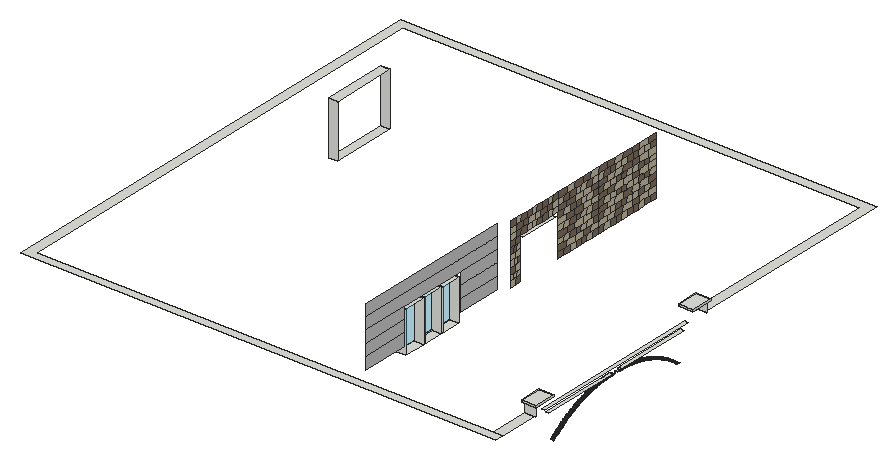
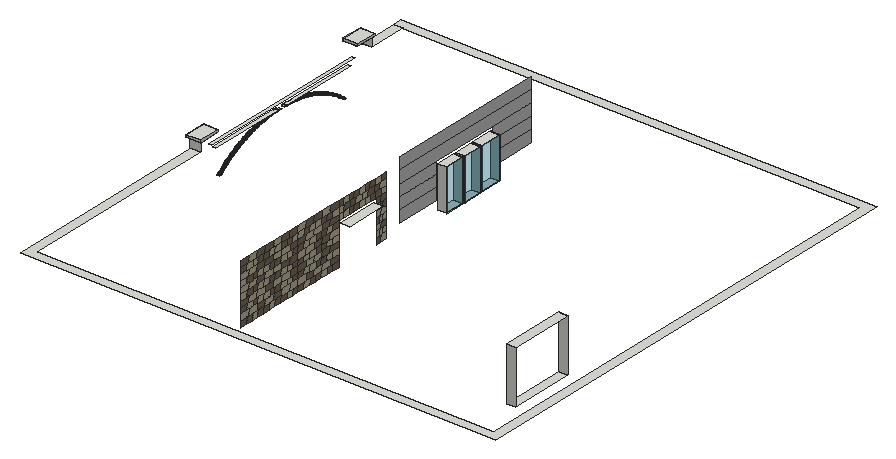
# SketchUp Ruby script. Lengths in inches.
U = 1.inch
M = Sketchup.active_model
def pt(a) = Geom::Point3d.new(a.map { |v| v * U })
def face(e, loops, mat)
  f = e.add_face(loops[0].map { |a| pt(a) })
  loops[1..].each { |l| e.add_face(l.map { |a| pt(a) }).erase! }
  f.material = f.back_material = mat if mat
  f
end
# faces: each face lists its corners as indices into pts; further lists are holes
def faces(e, pts, list, mat = nil) = list.each { |f| face(e, (f[0].is_a?(Array) ? f : [f]).map { |l| l.map { |i| pts[i] } }, mat) }
# xy, xz, yz: faces in a plane at the given z, y or x. An outline is a flat list of corners, or four numbers for a rectangle; further outlines are holes
def ring(l) = l.size == 4 ? [[l[0], l[1]], [l[2], l[1]], [l[2], l[3]], [l[0], l[3]]] : l.each_slice(2).to_a
def flat(e, list, mat, &to3) = list.each { |f| face(e, (f[0].is_a?(Array) ? f : [f]).map { |l| ring(l).map { |u, v| to3.(u, v) } }, mat) }
def xy(e, z, list, mat = nil) = flat(e, list, mat) { |x, y| [x, y, z] }
def xz(e, y, list, mat = nil) = flat(e, list, mat) { |x, z| [x, y, z] }
def yz(e, x, list, mat = nil) = flat(e, list, mat) { |y, z| [x, y, z] }
def lines(e, pts, list) = list.each { |a, b| e.add_line(pt(pts[a]), pt(pts[b])) }
# prism: a flat outline (further loops are holes) pulled along v
def prism(e, loops, v, mat = nil)
  f = face(e, loops, mat); d = Geom::Vector3d.new(v.map { |x| x * U })
  f.pushpull(f.normal.samedirection?(d) ? d.length : -d.length)
end
def box(e, o, s, mat = nil) = prism(e, [[o, [o[0] + s[0], o[1], o[2]], [o[0] + s[0], o[1] + s[1], o[2]], [o[0], o[1] + s[1], o[2]]]], [0, 0, s[2]], mat)
def at(x, y, z, deg = 0) = Geom::Transformation.translation(pt([x, y, z])) * Geom::Transformation.rotation(ORIGIN, Z_AXIS, deg.degrees)
def axes(o, x, y, z) = Geom::Transformation.new([*x, 0, *y, 0, *z, 0, *pt(o).to_a, 1])
def part(name) = M.definitions.add(name)
# library, detail: a bought-in or finely detailed component or shape, given as its bounding box
def library(name, o, s) = part(name).tap { |d| box(d.entities, o, s) }
def detail(e, o, s) = box(e.add_group.entities, o, s)
def put(e, d, t, mat = nil) = e.add_instance(d, t).tap { |i| i.material = mat if mat }
def group(e, t, mat = nil) = e.add_group.tap { |g| g.transformation = t; g.material = mat if mat }.entities
root = M.entities
M.materials.add("Brick_05_1K").color = [195, 185, 161]
M.materials.add("Brick_20_1K1").color = [126, 109, 93]
M.materials.add("Glass_Basic_01").color = [33, 150, 186]
M.materials["Glass_Basic_01"].alpha = 0.4
M.materials.add("M02_Ash_Whisper").color = [196, 196, 196]
M.materials.add("ThomThom - Buttons1").color = [48, 49, 53]
xy(root,63,[[294,108,303,130],[57,318,66,384]])
xy(root,86.9,[[474,151,477,153.9],[474,158.1,477,161]])
xy(root,88,[[474,71,477,151],[474,161,477,241]])
xy(root,93,[[474,66,477,246]])
xy(root,96,[[0,0,480,0,480,9,9,9,9,471,471,471,471,264,480,264,480,480,0,480],[471,9,480,48]])
xy(root,105,[[294,108,303,130],[294,255,303,297]])
xy(root,106,[[469,46,484,48],[469,48,471,68],[482,48,484,66],[471,66,480,68],[480,66,484,68],
  [469,244,484,246],[469,246,471,264],[482,246,484,264],[469,264,480,266],[480,264,484,266]])
xy(root,108,[[469,46,484,68],[469,244,484,266]])
xy(root,117,[[57,318,66,384]])
xz(root,46,[[469,106,484,108]])
xz(root,48,[[471,96,482,106]])
xz(root,68,[[469,106,484,108]])
xz(root,108,[[294,63,303,105]])
xz(root,130,[[294,63,303,105]])
xz(root,132.01,[[294,62.88,303,104.88]])
xz(root,152,[[294,63,303,105]])
xz(root,154.01,[[294,62.88,303,104.88]])
xz(root,174,[[294,63,303,105]])
xz(root,244,[[469,106,484,108]])
xz(root,264,[[471,96,482,106]])
xz(root,266,[[469,106,484,108]])
xz(root,318,[[57,63,66,117]])
xz(root,384,[[57,63,66,117]])
yz(root,294,[[132.01,62.88,152,63,152,62.88],[154.01,62.88,174,63,174,62.88],[132.01,104.88,132.01,105,152,105],[154.01,104.88,154.01,105,174,105]])
yz(root,294,[[132.01,62.88,132.01,104.88,152,105,152,63],[154.01,62.88,154.01,104.88,174,105,174,63],[108,63,130,105]],"Glass_Basic_01")
yz(root,303,[[240,66,246,72],[314.47,66,321.71,72],[336.18,66,343.41,72],[357.88,66,365.12,72],[379.59,66,386.82,72],
  [401.29,66,408.53,72],[240,72,244,78],[244,72,248,78],[248,72,252,78],[310.25,72,320.5,78],
  [320.5,72,330.75,78],[341,72,351.25,78],[351.25,72,361.5,78],[361.5,72,371.75,78],[382,72,392.25,78],
  [402.5,72,412.75,78],[412.75,72,423,78],[246,78,252,84],[300,78,307.24,84],[307.24,78,314.47,84],
  [328.94,78,336.18,84],[336.18,78,343.41,84],[357.88,78,365.12,84],[365.12,78,372.35,84],[386.82,78,394.06,84],
  [394.06,78,401.29,84],[408.53,78,415.76,84],[240,84,244,90],[244,84,248,90],[320.5,84,330.75,90],
  [330.75,84,341,90],[361.5,84,371.75,90],[371.75,84,382,90],[392.25,84,402.5,90],[402.5,84,412.75,90],
  [240,90,246,96],[246,90,252,96],[300,90,307.24,96],[307.24,90,314.47,96],[328.94,90,336.18,96],
  [336.18,90,343.41,96],[357.88,90,365.12,96],[365.12,90,372.35,96],[386.82,90,394.06,96],[394.06,90,401.29,96],
  [415.76,90,423,96],[248,96,252,102],[300,96,310.25,102],[330.75,96,341,102],[341,96,351.25,102],
  [371.75,96,382,102],[382,96,392.25,102],[402.5,96,412.75,102],[412.75,96,423,102],[307.24,102,314.47,108],
  [328.94,102,336.18,108],[336.18,102,343.41,108],[357.88,102,365.12,108],[365.12,102,372.35,108],[386.82,102,394.06,108],
  [394.06,102,401.29,108],[415.76,102,423,108],[240,108,246.67,114],[260,108,266.67,114],[266.67,108,273.33,114],
  [286.67,108,293.33,114],[293.33,108,300,114],[320.5,108,330.75,114],[330.75,108,341,114],[361.5,108,371.75,114],
  [371.75,108,382,114],[402.5,108,412.75,114],[412.75,108,423,114],[240,114,247.5,120],[262.5,114,270,120],
  [270,114,277.5,120],[292.5,114,300,120],[300,114,307.24,120],[321.71,114,328.94,120],[328.94,114,336.18,120],
  [343.41,114,350.65,120],[350.65,114,357.88,120],[372.35,114,379.59,120],[379.59,114,386.82,120],[401.29,114,408.53,120],
  [408.53,114,415.76,120],[246.67,120,253.33,126],[266.67,120,273.33,126],[286.67,120,293.33,126],[310.25,120,320.5,126],
  [341,120,351.25,126],[371.75,120,382,126],[402.5,120,412.75,126]],"Brick_05_1K")
yz(root,303,[[246,66,252,72],[300,66,307.24,72],[307.24,66,314.47,72],[321.71,66,328.94,72],[328.94,66,336.18,72],
  [343.41,66,350.65,72],[350.65,66,357.88,72],[365.12,66,372.35,72],[372.35,66,379.59,72],[386.82,66,394.06,72],
  [394.06,66,401.29,72],[408.53,66,415.76,72],[415.76,66,423,72],[300,72,310.25,78],[330.75,72,341,78],
  [371.75,72,382,78],[392.25,72,402.5,78],[240,78,246,84],[314.47,78,321.71,84],[321.71,78,328.94,84],
  [343.41,78,350.65,84],[350.65,78,357.88,84],[372.35,78,379.59,84],[379.59,78,386.82,84],[401.29,78,408.53,84],
  [415.76,78,423,84],[248,84,252,90],[300,84,310.25,90],[310.25,84,320.5,90],[341,84,351.25,90],
  [351.25,84,361.5,90],[382,84,392.25,90],[412.75,84,423,90],[314.47,90,321.71,96],[321.71,90,328.94,96],
  [343.41,90,350.65,96],[350.65,90,357.88,96],[372.35,90,379.59,96],[379.59,90,386.82,96],[401.29,90,408.53,96],
  [408.53,90,415.76,96],[240,96,244,102],[244,96,248,102],[310.25,96,320.5,102],[320.5,96,330.75,102],
  [351.25,96,361.5,102],[361.5,96,371.75,102],[392.25,96,402.5,102],[240,102,246,108],[246,102,252,108],
  [300,102,307.24,108],[314.47,102,321.71,108],[321.71,102,328.94,108],[343.41,102,350.65,108],[350.65,102,357.88,108],
  [372.35,102,379.59,108],[379.59,102,386.82,108],[401.29,102,408.53,108],[408.53,102,415.76,108],[246.67,108,253.33,114],
  [253.33,108,260,114],[273.33,108,280,114],[280,108,286.67,114],[300,108,310.25,114],[310.25,108,320.5,114],
  [341,108,351.25,114],[351.25,108,361.5,114],[382,108,392.25,114],[392.25,108,402.5,114],[247.5,114,255,120],
  [255,114,262.5,120],[277.5,114,285,120],[285,114,292.5,120],[307.24,114,314.47,120],[314.47,114,321.71,120],
  [336.18,114,343.41,120],[357.88,114,365.12,120],[365.12,114,372.35,120],[386.82,114,394.06,120],[394.06,114,401.29,120],
  [415.76,114,423,120],[240,120,246.67,126],[253.33,120,260,126],[260,120,266.67,126],[273.33,120,280,126],
  [280,120,286.67,126],[293.33,120,300,126],[300,120,310.25,126],[320.5,120,330.75,126],[330.75,120,341,126],
  [351.25,120,361.5,126],[361.5,120,371.75,126],[382,120,392.25,126],[392.25,120,402.5,126],[412.75,120,423,126]],"Brick_20_1K1")
yz(root,303,[[57,72,105,84],[177,72,222,84],[57,84,105,96],[177,84,222,96],[57,96,105,108],
  [177,96,222,108],[57,108,222,120],[57,120,222,132]],"M02_Ash_Whisper")
yz(root,469,[[46,106,68,108],[244,106,266,108]])
yz(root,477,[[151,88,154,88,152.18,88.01]])
yz(root,484,[[46,106,68,108],[244,106,266,108]])
p = [[477,76.49,60.8],[477,77.9,61.95],[474,77.9,61.95],[474,76.49,60.8],[477,234.1,61.95],[477,235.51,60.8],
  [474,235.51,60.8],[474,234.1,61.95],[477,78.59,61.09],[477,78.42,60.95],[474,78.42,60.95],[474,78.59,61.09],
  [477,233.58,60.95],[477,233.41,61.09],[474,233.41,61.09],[474,233.58,60.95],[477,80.01,62.21],[474,80.01,62.21],
  [477,231.99,62.21],[474,231.99,62.21],[477,78.32,62.28],[474,78.32,62.28],[477,232.66,63.08],[474,232.66,63.08],
  [477,81.45,63.3],[474,81.45,63.3],[477,230.55,63.3],[474,230.55,63.3],[477,79.34,63.08],[474,79.34,63.08],
  [303,132.01,62.88],[303,152,63],[294,152,63],[294,132.01,62.88],[303,154.01,62.88],[303,174,63],
  [294,174,63],[294,154.01,62.88],[477,80.79,64.18],[474,80.79,64.18],[477,231.21,64.18],[474,231.21,64.18],
  [477,82.9,64.37],[474,82.9,64.37],[477,229.1,64.37],[474,229.1,64.37],[477,82.25,65.26],[474,82.25,65.26],
  [477,229.75,65.26],[474,229.75,65.26],[477,82.95,64.4],[474,82.95,64.4],[477,229.05,64.4],[474,229.05,64.4],
  [477,84.37,65.42],[477,83.15,64.55],[474,83.15,64.55],[474,84.37,65.42],[477,228.85,64.55],[477,227.63,65.42],
  [474,227.63,65.42],[474,228.85,64.55],[477,83.05,65.83],[474,83.05,65.83],[477,228.26,66.32],[474,228.26,66.32],
  [477,85.86,66.45],[474,85.86,66.45],[477,226.14,66.45],[474,226.14,66.45],[477,83.74,66.32],[474,83.74,66.32],
  [477,85.24,67.36],[474,85.24,67.36],[477,226.76,67.36],[474,226.76,67.36],[477,87.36,67.45],[474,87.36,67.45],
  [477,224.64,67.45],[474,224.64,67.45],[477,86.75,68.37],[474,86.75,68.37],[477,225.25,68.37],[474,225.25,68.37],
  [477,87.68,67.66],[474,87.68,67.66],[477,224.32,67.66],[474,224.32,67.66],[477,88.875,68.43],[477,87.88,67.79],
  [474,87.88,67.79],[474,88.875,68.43],[477,224.12,67.79],[477,223.125,68.43],[474,223.125,68.43],[474,224.12,67.79],
  [477,87.78,69.03],[474,87.78,69.03],[477,90.41,69.39],[474,90.41,69.39],[477,221.59,69.39],[474,221.59,69.39],
  [477,223.72,69.36],[474,223.72,69.36],[477,88.28,69.36],[474,88.28,69.36],[477,89.83,70.33],[474,89.83,70.33],
  [477,91.95,70.32],[474,91.95,70.32],[477,220.05,70.32],[474,220.05,70.32],[477,222.17,70.33],[474,222.17,70.33],
  [477,91.39,71.27],[474,91.39,71.27],[477,92.41,70.59],[474,92.41,70.59],[477,219.59,70.59],[474,219.59,70.59],
  [477,220.61,71.27],[474,220.61,71.27],[477,93.51,71.23],[477,92.61,70.71],[474,92.61,70.71],[474,93.51,71.23],
  [477,219.39,70.71],[477,218.49,71.23],[474,218.49,71.23],[474,219.39,70.71],[477,95.09,72.12],[474,95.09,72.12],
  [477,216.91,72.12],[474,216.91,72.12],[477,92.51,71.92],[474,92.51,71.92],[477,219.03,72.1875],[474,219.03,72.1875],
  [477,92.97,72.1875],[474,92.97,72.1875],[477,96.67,72.98],[474,96.67,72.98],[477,215.33,72.98],[474,215.33,72.98],
  [477,94.55,73.08],[474,94.55,73.08],[477,217.45,73.08],[474,217.45,73.08],[477,97.14,73.23],[474,97.14,73.23],
  [477,214.86,73.23],[474,214.86,73.23],[477,96.16,73.95],[474,96.16,73.95],[477,215.84,73.95],[474,215.84,73.95],
  [477,98.27,73.82],[477,97.34,73.33],[474,97.34,73.33],[474,98.27,73.82],[477,214.66,73.33],[477,213.73,73.82],
  [474,213.73,73.82],[474,214.66,73.33],[477,99.89,74.63],[474,99.89,74.63],[477,212.11,74.63],[474,212.11,74.63],
  [477,97.24,74.52],[474,97.24,74.52],[477,214.23,74.8],[474,214.23,74.8],[477,97.77,74.8],[474,97.77,74.8],
  [477,101.51,75.42],[474,101.51,75.42],[477,210.49,75.42],[474,210.49,75.42],[477,99.4,75.62],[474,99.4,75.62],
  [477,212.6,75.62],[474,212.6,75.62],[477,101.87,75.59],[474,101.87,75.59],[477,210.13,75.59],[474,210.13,75.59],
  [477,101.04,76.42],[474,101.04,76.42],[477,210.96,76.42],[474,210.96,76.42],[477,103.15,76.1875],[477,102.07,75.68],
  [474,102.07,75.68],[474,103.15,76.1875],[477,209.93,75.68],[477,208.85,76.1875],[474,208.85,76.1875],[474,209.93,75.68],
  [477,104.8,76.93],[474,104.8,76.93],[477,207.2,76.93],[474,207.2,76.93],[477,101.97,76.85],[474,101.97,76.85],
  [477,209.31,77.1875],[474,209.31,77.1875],[477,102.69,77.1875],[474,102.69,77.1875],[477,106.45,77.64],[474,106.45,77.64],
  [477,205.55,77.64],[474,205.55,77.64],[477,104.35,77.93],[474,104.35,77.93],[477,207.65,77.93],[474,207.65,77.93],
  [477,106.6,77.7],[474,106.6,77.7],[477,205.4,77.7],[474,205.4,77.7],[477,108.125,78.33],[477,106.8,77.78],
  [474,106.8,77.78],[474,108.125,78.33],[477,205.2,77.78],[477,203.875,78.33],[474,203.875,78.33],[474,205.2,77.78],
  [477,106.03,78.65],[474,106.03,78.65],[477,205.97,78.65],[474,205.97,78.65],[477,109.81,78.99],[474,109.81,78.99],
  [477,202.19,78.99],[474,202.19,78.99],[477,106.7,78.93],[474,106.7,78.93],[477,204.29,79.35],[474,204.29,79.35],
  [477,107.71,79.35],[474,107.71,79.35],[477,111.33,79.5625],[474,111.33,79.5625],[477,200.67,79.5625],[474,200.67,79.5625],
  [477,109.41,80.02],[474,109.41,80.02],[477,202.59,80.02],[474,202.59,80.02],[477,113.2,80.24],[477,111.53,79.64],
  [474,111.53,79.64],[474,113.2,80.24],[477,200.47,79.64],[477,198.8,80.24],[474,198.8,80.24],[474,200.47,79.64],
  [477,111.12,80.66],[474,111.12,80.66],[477,200.88,80.66],[474,200.88,80.66],[477,114.9,80.82],[474,114.9,80.82],
  [477,197.1,80.82],[474,197.1,80.82],[477,111.43,80.77],[474,111.43,80.77],[477,199.17,81.28],[474,199.17,81.28],
  [477,112.83,81.28],[474,112.83,81.28],[477,116.06,81.2],[474,116.06,81.2],[477,195.94,81.2],[474,195.94,81.2],
  [477,114.56,81.87],[474,114.56,81.87],[477,116.62,81.38],[477,116.26,81.26],[474,116.26,81.26],[474,116.62,81.38],
  [477,195.74,81.26],[477,195.38,81.38],[474,195.38,81.38],[474,195.74,81.26],[477,197.44,81.87],[474,197.44,81.87],
  [477,118.35,81.91],[474,118.35,81.91],[477,193.65,81.91],[474,193.65,81.91],[477,116.16,82.39],[474,116.16,82.39],
  [477,120.08,82.42],[474,120.08,82.42],[477,191.92,82.42],[474,191.92,82.42],[477,195.71,82.43],[474,195.71,82.43],
  [477,116.29,82.43],[474,116.29,82.43],[477,118.03,82.97],[474,118.03,82.97],[477,120.79,82.61],[474,120.79,82.61],
  [477,191.21,82.61],[474,191.21,82.61],[477,193.97,82.97],[474,193.97,82.97],[477,121.82,82.9],[477,120.99,82.67],
  [474,120.99,82.67],[474,121.82,82.9],[477,191.01,82.67],[477,190.18,82.9],[474,190.18,82.9],[474,191.01,82.67],
  [477,123.57,83.35],[474,123.57,83.35],[477,188.43,83.35],[474,188.43,83.35],[477,119.78,83.48],[474,119.78,83.48],
  [477,192.22,83.48],[474,192.22,83.48],[477,125.33,83.78],[474,125.33,83.78],[477,186.67,83.78],[474,186.67,83.78],
  [477,120.89,83.78],[474,120.89,83.78],[477,190.46,83.96],[474,190.46,83.96],[477,121.54,83.96],[474,121.54,83.96],
  [477,125.52,83.82],[474,125.52,83.82],[477,186.48,83.82],[474,186.48,83.82],[477,127.09,84.18],[477,125.72,83.87],
  [474,125.72,83.87],[474,127.09,84.18],[477,186.28,83.87],[477,184.91,84.18],[474,184.91,84.18],[474,186.28,83.87],
  [477,123.3,84.42],[474,123.3,84.42],[477,188.7,84.42],[474,188.7,84.42],[477,128.86,84.55],[474,128.86,84.55],
  [477,183.14,84.55],[474,183.14,84.55],[477,125.08,84.85],[474,125.08,84.85],[477,186.92,84.85],[474,186.92,84.85],
  [477,130.25,84.82],[474,130.25,84.82],[477,181.75,84.82],[474,181.75,84.82],[477,125.62,84.97],[474,125.62,84.97],
  [477,185.15,85.25],[474,185.15,85.25],[477,130.63,84.9],[477,130.45,84.86],[474,130.45,84.86],[474,130.63,84.9],
  [477,132.41,85.21],[474,132.41,85.21],[477,181.37,84.9],[477,179.59,85.21],[474,179.59,85.21],[474,181.37,84.9],
  [477,181.55,84.86],[474,181.55,84.86],[477,126.85,85.25],[474,126.85,85.25],[477,134.1875,85.51],[474,134.1875,85.51],
  [477,177.8125,85.51],[474,177.8125,85.51],[477,128.64,85.63],[474,128.64,85.63],[477,183.36,85.63],[474,183.36,85.63],
  [477,134.98,85.62],[474,134.98,85.62],[477,177.02,85.62],[474,177.02,85.62],[477,130.35,85.96],[474,130.35,85.96],
  [477,181.57,85.98],[474,181.57,85.98],[477,135.98,85.77],[477,135.18,85.65],[474,135.18,85.65],[474,135.98,85.77],
  [477,176.82,85.65],[477,176.02,85.77],[474,176.02,85.77],[474,176.82,85.65],[477,137.77,86.01],[474,137.77,86.01],
  [477,174.23,86.01],[474,174.23,86.01],[477,130.43,85.98],[474,130.43,85.98],[477,132.22,86.3],[474,132.22,86.3],
  [477,139.56,86.22],[474,139.56,86.22],[477,172.44,86.22],[474,172.44,86.22],[477,179.78,86.3],[474,179.78,86.3],
  [477,139.71,86.23],[474,139.71,86.23],[477,172.29,86.23],[474,172.29,86.23],[477,134.02,86.59],[474,134.02,86.59],
  [477,141.36,86.4],[477,139.91,86.25],[474,139.91,86.25],[474,141.36,86.4],[477,172.09,86.25],[477,170.64,86.4],
  [474,170.64,86.4],[474,172.09,86.25],[477,177.98,86.59],[474,177.98,86.59],[477,143.16,86.55],[474,143.16,86.55],
  [477,168.84,86.55],[474,168.84,86.55],[477,135.08,86.75],[474,135.08,86.75],[477,144.44,86.64],[474,144.44,86.64],
  [477,167.56,86.64],[474,167.56,86.64],[477,176.18,86.86],[474,176.18,86.86],[477,135.82,86.86],[474,135.82,86.86],
  [477,144.96,86.68],[477,144.64,86.66],[474,144.64,86.66],[474,144.96,86.68],[477,146.76,86.78],[474,146.76,86.78],
  [477,167.04,86.68],[477,165.24,86.78],[474,165.24,86.78],[474,167.04,86.68],[477,167.36,86.66],[474,167.36,86.66],
  [477,148.57,86.85],[474,148.57,86.85],[477,149.17,86.86],[474,149.17,86.86],[477,163.43,86.85],[477,162.83,86.86],
  [474,162.83,86.86],[474,163.43,86.85],[477,137.63,87.1],[474,137.63,87.1],[477,150.37,86.89],[477,149.37,86.87],
  [474,149.37,86.87],[474,150.37,86.89],[477,151,86.9],[474,151,86.9],[477,161.63,86.89],[477,161,86.9],
  [474,161,86.9],[474,161.63,86.89],[477,162.63,86.87],[474,162.63,86.87],[477,174.37,87.1],[474,174.37,87.1],
  [477,139.44,87.31],[474,139.44,87.31],[477,172.56,87.31],[474,172.56,87.31],[477,141.25,87.49],[474,141.25,87.49],
  [477,170.75,87.49],[474,170.75,87.49],[477,143.07,87.65],[474,143.07,87.65],[477,168.93,87.65],[474,168.93,87.65],
  [477,144.89,87.78],[474,144.89,87.78],[477,167.11,87.78],[474,167.11,87.78],[477,146.71,87.875],[474,146.71,87.875],
  [477,165.29,87.875],[474,165.29,87.875],[477,148.53,87.95],[474,148.53,87.95],[477,150.35,87.99],[474,150.35,87.99],
  [477,161.65,87.99],[477,163.47,87.95],[474,163.47,87.95],[474,161.65,87.99],[477,151,88],[474,151,88],
  [477,161,88],[474,161,88],[303,152,105],[303,132.01,104.88],[294,132.01,104.88],[294,152,105],
  [303,174,105],[303,154.01,104.88],[294,154.01,104.88],[294,174,105],[477,149.27,86.97],[477,149.27,87]]
faces(root,p,[[0,1,2,3],[4,5,6,7],[1,20,21,2],[22,4,7,23],[20,28,29,21],[28,38,39,29],[40,22,23,41],[38,46,47,39],
  [48,40,41,49],[46,62,63,47],[64,48,49,65],[62,70,71,63],[70,72,73,71],[74,64,65,75],[72,80,81,73],[82,74,75,83],
  [80,96,97,81],[102,82,83,103],[96,104,105,97],[104,106,107,105],[112,102,103,113],[106,114,115,107],[120,112,113,121],[114,134,135,115],
  [136,120,121,137],[134,138,139,135],[138,144,145,139],[146,136,137,147],[144,152,153,145],[154,146,147,155],[152,168,169,153],[170,154,155,171],
  [168,172,173,169],[172,178,179,173],[180,170,171,181],[178,186,187,179],[188,180,181,189],[186,202,203,187],[204,188,189,205],[202,206,207,203],
  [206,212,213,207],[214,204,205,215],[212,228,229,213],[230,214,215,231],[228,236,237,229],[238,230,231,239],[236,240,241,237],[240,246,247,241],
  [248,238,239,249],[246,258,259,247],[260,248,249,261],[258,266,267,259],[268,260,261,269],[266,270,271,267],[270,276,277,271],[286,268,269,287],
  [276,292,293,277],[298,286,287,299],[292,300,301,293],[300,302,303,301],[308,298,299,309],[302,322,323,303],[324,308,309,325],[322,330,331,323],
  [332,324,325,333],[330,334,335,331],[334,348,349,335],[350,332,333,351],[348,356,357,349],[358,350,351,359],[356,364,365,357],[366,358,359,367],
  [364,380,381,365],[380,386,387,381],[388,366,367,389],[386,394,395,387],[396,388,389,397],[394,410,411,395],[410,412,413,411],[418,396,397,419],
  [412,424,425,413],[434,418,419,435],[424,440,441,425],[446,434,435,447],[440,448,449,441],[448,470,471,449],[484,446,447,485],[470,486,487,471],
  [488,484,485,489],[486,490,491,487],[492,488,489,493],[490,494,495,491],[496,492,493,497],[494,498,499,495],[500,496,497,501],[498,502,503,499],
  [504,500,501,505],[502,506,507,503],[506,508,509,507],[510,511,512,513],[511,504,505,512],[508,514,515,509]],"ThomThom - Buttons1")
faces(root,p,[[8,9,10,11],[12,13,14,15],[16,8,11,17],[13,18,19,14],[24,16,17,25],[18,26,27,19],[30,31,32,33],[34,35,36,37],
  [42,24,25,43],[26,44,45,27],[50,42,43,51],[44,52,53,45],[54,55,56,57],[58,59,60,61],[66,54,57,67],[59,68,69,60],
  [76,66,67,77],[68,78,79,69],[84,76,77,85],[78,86,87,79],[88,89,90,91],[92,93,94,95],[98,88,91,99],[93,100,101,94],
  [108,98,99,109],[100,110,111,101],[116,108,109,117],[110,118,119,111],[122,123,124,125],[126,127,128,129],[130,122,125,131],[127,132,133,128],
  [140,130,131,141],[132,142,143,133],[148,140,141,149],[142,150,151,143],[156,157,158,159],[160,161,162,163],[164,156,159,165],[161,166,167,162],
  [174,164,165,175],[166,176,177,167],[182,174,175,183],[176,184,185,177],[190,191,192,193],[194,195,196,197],[198,190,193,199],[195,200,201,196],
  [208,198,199,209],[200,210,211,201],[216,208,209,217],[210,218,219,211],[220,221,222,223],[224,225,226,227],[232,220,223,233],[225,234,235,226],
  [242,232,233,243],[234,244,245,235],[250,251,252,253],[254,255,256,257],[262,250,253,263],[255,264,265,256],[272,262,263,273],[264,274,275,265],
  [278,279,280,281],[282,283,284,285],[288,278,281,289],[283,290,291,284],[294,288,289,295],[290,296,297,291],[304,294,295,305],[296,306,307,297],
  [310,311,312,313],[314,315,316,317],[318,310,313,319],[315,320,321,316],[326,318,319,327],[320,328,329,321],[336,326,327,337],[328,338,339,329],
  [340,341,342,343],[344,345,346,347],[352,340,343,353],[345,354,355,346],[360,352,353,361],[354,362,363,355],[368,369,370,371],[372,368,371,373],
  [374,375,376,377],[378,374,377,379],[382,372,373,383],[375,384,385,376],[390,382,383,391],[384,392,393,385],[398,399,400,401],[402,403,404,405],
  [406,398,401,407],[403,408,409,404],[414,406,407,415],[408,416,417,409],[420,414,415,421],[416,422,423,417],[426,427,428,429],[430,431,432,433],
  [436,426,429,437],[431,438,439,432],[442,436,437,443],[438,444,445,439],[450,451,452,453],[454,450,453,455],[456,457,458,459],[460,456,459,461],
  [462,454,455,463],[464,462,463,465],[466,467,468,469],[457,466,469,458],[472,473,474,475],[476,472,475,477],[478,479,480,481],[482,478,481,483],
  [516,510,513,517],[518,519,520,521],[522,523,524,525]])
lines(root,p,[[526,527]])
